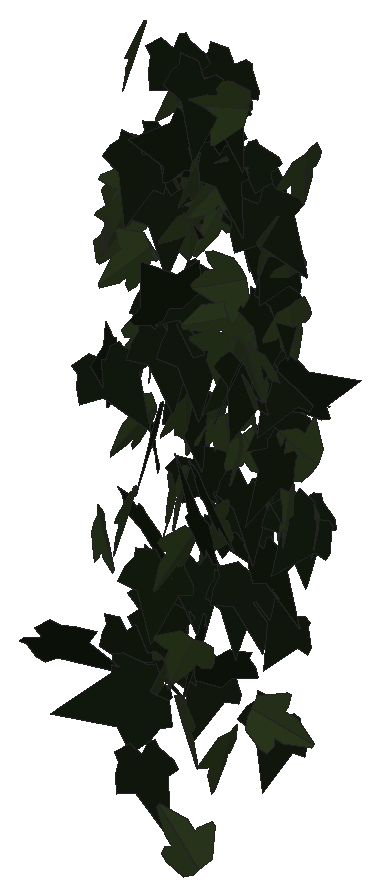
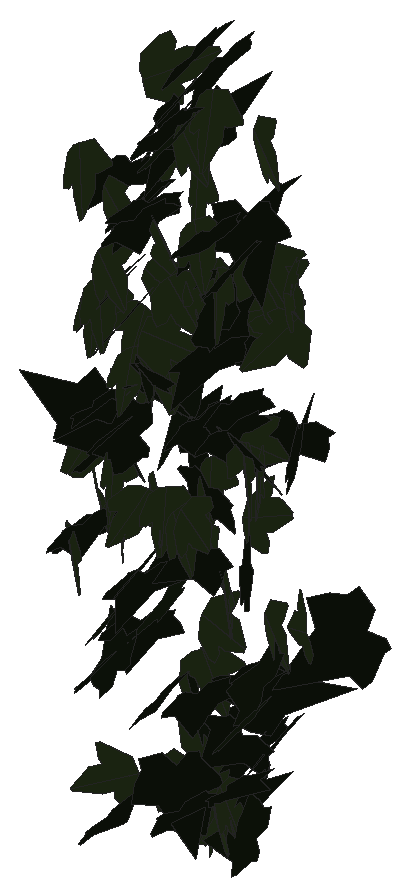
# SketchUp Ruby script. Lengths in inches.
U = 1.inch
M = Sketchup.active_model
def pt(a) = Geom::Point3d.new(a.map { |v| v * U })
def face(e, loops, mat)
  f = e.add_face(loops[0].map { |a| pt(a) })
  loops[1..].each { |l| e.add_face(l.map { |a| pt(a) }).erase! }
  f.material = f.back_material = mat if mat
  f
end
# faces: each face lists its corners as indices into pts; further lists are holes
def faces(e, pts, list, mat = nil) = list.each { |f| face(e, (f[0].is_a?(Array) ? f : [f]).map { |l| l.map { |i| pts[i] } }, mat) }
# xy, xz, yz: faces in a plane at the given z, y or x. An outline is a flat list of corners, or four numbers for a rectangle; further outlines are holes
def ring(l) = l.size == 4 ? [[l[0], l[1]], [l[2], l[1]], [l[2], l[3]], [l[0], l[3]]] : l.each_slice(2).to_a
def flat(e, list, mat, &to3) = list.each { |f| face(e, (f[0].is_a?(Array) ? f : [f]).map { |l| ring(l).map { |u, v| to3.(u, v) } }, mat) }
def xy(e, z, list, mat = nil) = flat(e, list, mat) { |x, y| [x, y, z] }
def xz(e, y, list, mat = nil) = flat(e, list, mat) { |x, z| [x, y, z] }
def yz(e, x, list, mat = nil) = flat(e, list, mat) { |y, z| [x, y, z] }
def lines(e, pts, list) = list.each { |a, b| e.add_line(pt(pts[a]), pt(pts[b])) }
# prism: a flat outline (further loops are holes) pulled along v
def prism(e, loops, v, mat = nil)
  f = face(e, loops, mat); d = Geom::Vector3d.new(v.map { |x| x * U })
  f.pushpull(f.normal.samedirection?(d) ? d.length : -d.length)
end
def box(e, o, s, mat = nil) = prism(e, [[o, [o[0] + s[0], o[1], o[2]], [o[0] + s[0], o[1] + s[1], o[2]], [o[0], o[1] + s[1], o[2]]]], [0, 0, s[2]], mat)
def at(x, y, z, deg = 0) = Geom::Transformation.translation(pt([x, y, z])) * Geom::Transformation.rotation(ORIGIN, Z_AXIS, deg.degrees)
def axes(o, x, y, z) = Geom::Transformation.new([*x, 0, *y, 0, *z, 0, *pt(o).to_a, 1])
def part(name) = M.definitions.add(name)
# library, detail: a bought-in or finely detailed component or shape, given as its bounding box
def library(name, o, s) = part(name).tap { |d| box(d.entities, o, s) }
def detail(e, o, s) = box(e.add_group.entities, o, s)
def put(e, d, t, mat = nil) = e.add_instance(d, t).tap { |i| i.material = mat if mat }
def group(e, t, mat = nil) = e.add_group.tap { |g| g.transformation = t; g.material = mat if mat }.entities
root = M.entities
M.materials.add("efeu1").color = [18, 25, 13]
M.materials.add("efeu2").color = [43, 57, 29]
c1 = part("ivyleaf_10")
p = [[0,0.5,-0.03],[-0.0625,2.02,-0.43],[-0.19,2.01,-0.46],[-0.54,1.05,-0.29],[-0.52,0.625,-0.18],[-0.83,0.76,-0.28],
  [-1.16,0.64,-0.33],[-1.15,0.33,-0.24],[-0.77,-0.39,0.02],[-0.3,-0.51,0.16],[0.04,-0.48,0.23],[-0.02,2.01,-0.4375],
  [-0.06,2.01,-0.43],[0.04,-0.49,0.23],[0.67,-0.49,0.14],[1.38,0.36,-0.2],[1.375,0.51,-0.24],[0.81,0.65,-0.19],
  [0.62,0.59,-0.15],[0.6,1.09,-0.28],[0.5,1.23,-0.31]]
faces(c1.entities,p,[[0,1,2,3,4,5,6,7,8,9,10],[11,12,0,13,14,15,16,17,18,19,20]],"efeu2")
c2 = part("ivyleaf_9")
p = [[1.54,2.16,1.25],[1.36,2.04,1.19],[-0.21,0.99,0.68],[-0.71,1.11,0.82],[-0.85,0.86,0.67],[-0.8,0.17,0.21],
  [-0.9,-0.01,0.1],[-0.67,-0.16,-0.02],[-0.08,-0.08,-0.05],[-0.03,-0.6,-0.4],[0.65,-0.88,-0.66],[0.83,-0.6,-0.49],
  [1.29,-0.42,-0.43],[1.8125,-0.07,-0.26],[1.21,0.44,0.15]]
faces(c2.entities,p,[[0,1,2,3,4,5,6,7,8,9,10,11,12,13,14]],"efeu1")
put(root,c1,axes([556.3125,126.64,275.13],[0.56401,-0.9853,0.35993],[0.15903,-0.32362,-1.13511],[1.03686,0.5856,-0.02169]))
put(root,c2,axes([555.64,127.46,252],[0.64718,-0.92448,0.49192],[0.30397,-0.38755,-1.12823],[1.00212,0.71459,0.02453]))
put(root,c2,axes([556.3,124.88,260.05],[-0.03943,-0.04675,1.18196],[-0.13609,-1.17459,-0.05099],[1.17503,-0.13761,0.03375]))
put(root,c2,axes([556.6,128.28,247.51],[-0.50318,-0.81706,0.39442],[-0.06975,-0.41484,-0.94836],[0.90459,-0.48648,0.14626]))
put(root,c1,axes([556.28,125.15,266.33],[-0.59657,-0.49919,-0.8205],[0.62688,0.52937,-0.77787],[0.72761,-0.86537,-0.00254]))
put(root,c1,axes([556.13,125.17,267.91],[0.21056,-0.52441,1.07679],[0.75537,-0.7903,-0.53259],[0.92946,0.76107,0.1889]))
put(root,c1,axes([556.57,125.68,253.55],[0.52615,-0.98515,0.36041],[0.17062,-0.31747,-1.11685],[1.03504,0.55312,0.0009]))
put(root,c1,axes([556.99,125.87,260.45],[0.40424,-0.52426,-0.91045],[-0.30448,0.8752,-0.63915],[1.00552,0.47579,0.17248]))
put(root,c1,axes([556.09,124.25,252.81],[0.35761,-0.2319,1.0365],[0.97534,-0.36128,-0.41734],[0.42049,1.03522,0.08653]))
put(root,c2,axes([556.02,127.48,245.26],[0.7752,-0.5989,0.50781],[0.39859,-0.31467,-0.97959],[0.67652,0.87165,-0.00473]))
put(root,c1,axes([556.99,124.93,267.99],[-0.02031,-0.99944,0.55469],[0.00222,-0.55481,-0.99957],[1.14305,-0.01668,0.01179]))
put(root,c2,axes([557.23,127.23,262.06],[-1.05217,0.06643,-0.22014],[0.21492,-0.08246,-1.05212],[-0.08175,-1.07179,0.06731]))
put(root,c1,axes([557.22,125.64,269.07],[-0.63028,-0.84539,0.58403],[-0.11789,-0.62113,-1.02631],[1.02072,-0.59375,0.2421]))
put(root,c1,axes([557.16,126.46,261.02],[0.64091,-0.76042,-0.6346],[-0.23557,0.61715,-0.97742],[0.96201,0.65773,0.18344]))
put(root,c2,axes([556.81,127.05,255.54],[-0.4046,0.41446,0.94509],[0.05844,-1.00431,0.46544],[1.03032,0.21972,0.34474]))
put(root,c1,axes([557.2,126.33,261.59],[0.37304,0.66662,-0.89608],[-0.40166,-0.80146,-0.76343],[-1.04212,0.54753,-0.02651]))
put(root,c2,axes([556.9375,127.43,249.51],[-0.09955,-0.87645,0.59303],[0.15035,-0.60132,-0.86346],[1.0475,0.00302,0.18029]))
put(root,c2,axes([556.86,127.77,269.95],[0.2655,-1.08538,0.06413],[0.01067,-0.06341,-1.11737],[1.08722,0.26567,-0.00469]))
put(root,c2,axes([557.11,127.61,262.68],[-0.11286,-1.0882,-0.13553],[0.02533,0.13362,-1.09398],[1.09631,-0.11511,0.01133]))
put(root,c1,axes([557.44,127.375,246.45],[0.16474,-0.9735,0.30647],[0.09722,-0.29406,-0.98633],[1.01596,0.18599,0.04469]))
put(root,c1,axes([557.375,125.68,257.94],[0.09628,-0.37219,1.11823],[0.27094,-1.08492,-0.38443],[1.14698,0.28752,-0.00306]))
put(root,c2,axes([557.87,125.52,270.79],[0.60279,0.64029,-0.79161],[-0.55902,-0.56074,-0.87923],[-0.85095,0.82193,0.01684]))
put(root,c2,axes([557.02,123.64,261.15],[-0.16084,-0.59584,-0.9611],[0.46324,0.85087,-0.60502],[1.03158,-0.47499,0.12184]))
put(root,c2,axes([557.15,124.82,247.8],[0.24998,-1.07113,0.17564],[0.04005,-0.17101,-1.09991],[1.0847,0.25317,0.00014]))
put(root,c1,axes([557.59,127.51,245.57],[0.59434,-0.90486,0.25286],[0.14863,-0.20489,-1.08253],[0.9277,0.61253,0.01143]))
put(root,c2,axes([557.77,126.07,245.24],[-0.22502,-0.61711,0.98012],[-0.35882,-0.91218,-0.65671],[1.10123,-0.42332,-0.01371]))
put(root,c1,axes([557.92,126.375,245.75],[0.44509,-0.9799,0.09472],[0.03724,-0.08711,-1.07624],[0.98376,0.44664,-0.00211]))
put(root,c1,axes([557.97,124.51,266.23],[-0.21681,-0.17831,1.10809],[0.12288,-1.12556,-0.15708],[1.1156,0.08933,0.23265]))
put(root,c2,axes([557.34,119.23,250.14],[1.22806,0.44859,0.46219],[0.43137,0.16613,-1.3074],[-0.47831,1.30159,0.00758]))
put(root,c1,axes([558.21,126.78,268.36],[0.79931,-0.48239,-0.64322],[-0.20259,0.75689,-0.81939],[0.77806,0.69263,0.44743]))
put(root,c2,axes([558.02,124.67,270.8125],[-0.11677,-1.08771,0.36615],[-0.02693,-0.36534,-1.0939],[1.14737,-0.11928,0.01159]))
put(root,c2,axes([558.15,125.9,250.85],[-0.38996,-1.00944,-0.1488],[0.0464,0.14159,-1.08212],[1.01929,-0.39264,-0.00767]))
put(root,c2,axes([557.87,125.95,248.41],[-0.24815,-0.42512,-1.00772],[0.80186,0.63202,-0.46408],[0.7438,-0.82319,0.16411]))
put(root,c1,axes([558.89,125.57,254.54],[0.40704,-0.65288,-0.73768],[-0.35175,0.64924,-0.76869],[0.92017,0.53699,0.03247]))
put(root,c2,axes([557.92,127.3,266.86],[0.14674,-0.48156,1.01776],[0.61545,-0.82516,-0.47917],[0.94285,0.61358,0.15438]))
put(root,c2,axes([558.28,127.41,270.79],[0.25732,-1.02174,-0.43615],[0.00733,0.44925,-1.0481],[1.11091,0.2337,0.10794]))
put(root,c2,axes([558.52,125.94,268.45],[-0.24771,-1.09137,-0.19604],[0.03207,0.19373,-1.11907],[1.10838,-0.24952,-0.01143]))
put(root,c1,axes([559.11,127.04,270.24],[-0.1522,-1.11281,-0.02709],[0.00219,0.02705,-1.12316],[1.11313,-0.15221,-0.00149]))
put(root,c2,axes([558.76,125.5,262.27],[-0.22177,-1.04022,-0.37124],[0.04911,0.36899,-1.06325],[1.10339,-0.2255,-0.0273]))
put(root,c2,axes([558.81,127.35,250.47],[-0.16845,-1.02661,-0.32116],[0.03345,0.31992,-1.04018],[1.07515,-0.1708,-0.01795]))
put(root,c1,axes([559.05,127.64,258.17],[-0.04841,-0.89408,0.60434],[0.20178,-0.60178,-0.87413],[1.06014,0.07371,0.19397]))
put(root,c2,axes([559.23,127.875,245.49],[-0.38874,-1.06838,0.09552],[-0.0348,-0.08898,-1.13691],[1.07208,-0.39029,-0.00227]))
put(root,c1,axes([559.46,127.74,257.78],[0.11033,-1.05731,0.12968],[0.00012,-0.13036,-1.06297],[1.06523,0.10952,-0.01331]))
put(root,c1,axes([559.5,125.63,259.18],[0.05269,-1.05707,-0.36706],[0.01665,0.36817,-1.05787],[1.11886,0.0443,0.03303]))
put(root,c1,axes([559.53,126.03,267.85],[-0.21648,-1.11946,-0.14462],[0.02582,0.14231,-1.14019],[1.12846,-0.21801,-0.00165]))
put(root,c2,axes([558.95,126.61,259.1],[-0.52797,-0.28013,-0.95176],[0.91114,0.28975,-0.59072],[0.39262,-1.04912,0.09099]))
put(root,c1,axes([559.49,125.63,252.64],[0.09184,-0.82512,0.77525],[0.08397,-0.77069,-0.83021],[1.12906,0.12443,-0.00132]))
put(root,c2,axes([559.47,124.67,264.29],[0.50512,0.44437,1.07602],[-0.78128,-0.74017,0.67244],[0.86306,-0.93011,-0.02104]))
put(root,c1,axes([559.86,127.48,267.76],[-0.57232,-0.80064,0.53157],[-0.1343,-0.54599,-0.96695],[0.9516,-0.55858,0.18323]))
put(root,c2,axes([559.14,126.02,264.75],[0.20337,-0.97242,-0.72905],[-0.00249,0.73885,-0.98619],[1.21536,0.16424,0.11997]))
put(root,c1,axes([559.28,125.79,244.57],[-0.71558,0.75391,-0.60071],[0.4061,-0.44273,-1.0394],[-0.87424,-0.82274,0.00887]))
put(root,c2,axes([560.06,127.09,246.68],[0.38264,0.88653,-0.68701],[-0.32498,-0.60711,-0.96444],[-1.07346,0.49981,0.04708]))
put(root,c2,axes([559.375,126.54,261.89],[-0.00036,-1.18226,-0.1288],[-0.01845,0.12879,-1.18212],[1.18911,0.00165,-0.01838]))
put(root,c1,axes([559.68,125.36,255.77],[0.66935,-0.79193,0.26859],[0.20283,-0.18001,-1.03623],[0.81127,0.6984,0.03747]))
put(root,c2,axes([560.41,122.02,247.41],[-0.10183,-0.7318,-1.20891],[-0.18243,-1.19509,0.73881],[-1.40133,0.20876,-0.00833]))
put(root,c1,axes([559.97,125.04,274.68],[-0.12336,-1.1411,-0.43764],[0.10773,0.428,-1.14633],[1.21739,-0.15351,0.0571]))
put(root,c1,axes([560.1,126.46,273.97],[0.17153,-1.09042,0.35447],[0.02946,-0.3541,-1.10356],[1.14621,0.17229,-0.02468]))
put(root,c2,axes([560,123.33,259.74],[-0.60976,0.22528,-0.94837],[0.8475,-0.43012,-0.64708],[-0.48156,-1.04221,0.06205]))
put(root,c2,axes([559.55,126.36,256.15],[-0.11195,-0.22365,-1.09413],[0.69957,0.84308,-0.24391],[0.87048,-0.7063,0.05531]))
put(root,c2,axes([559.91,124.53,276.53],[0.41084,-1.14036,-0.40828],[-0.11352,0.39297,-1.21185],[1.20591,0.4255,0.02502]))
put(root,c2,axes([560.0625,127.9375,274.06],[-0.02921,-0.96271,0.57528],[0.18384,-0.5718,-0.94756],[1.10633,0.0696,0.17264]))
put(root,c1,axes([560.73,124.9,271.09],[0.21692,-0.99031,-0.56397],[-0.06023,0.56333,-1.01236],[1.13805,0.21857,0.05392]))
put(root,c1,axes([560.65,127.02,258.11],[-0.36681,-1.00026,-0.15339],[0.16122,0.10331,-1.05922],[0.99903,-0.38394,0.11461]))
put(root,c2,axes([560.41,127.73,274.6],[-0.16549,-1.1053,0.19456],[-0.0353,-0.19144,-1.1176],[1.12173,-0.16909,-0.00647]))
put(root,c2,axes([560.7,125.32,248.85],[-0.68503,0.32815,-0.78247],[0.72694,-0.29168,-0.75874],[-0.4376,-0.99822,-0.03552]))
put(root,c2,axes([561.02,123.86,272.74],[-0.09089,-0.11257,1.15808],[-0.72882,-0.89998,-0.14468],[0.907,-0.73447,-0.00021]))
put(root,c2,axes([560.56,127.73,249.77],[0.09415,-1.01917,0.23102],[0.0438,-0.22791,-1.02327],[1.0441,0.10146,0.02209]))
put(root,c1,axes([561.48,123.59,249.29],[-0.82836,-0.49623,0.46274],[-0.38542,-0.25688,-0.96541],[0.55841,-0.91341,0.02011]))
put(root,c1,axes([560.43,127.26,269],[0.62028,-0.5236,-0.82353],[0.65692,-0.49759,0.81115],[-0.72169,-0.90297,0.03054]))
put(root,c2,axes([560.72,126.24,253.85],[0.82275,-0.5227,-0.42626],[-0.2102,0.44016,-0.94546],[0.64088,0.8154,0.23712]))
put(root,c1,axes([562.04,125.89,264.21],[-0.30228,-0.1415,1.10941],[-0.84916,-0.71885,-0.32306],[0.72783,-0.89745,0.08385]))
put(root,c2,axes([560.98,121.09,244.91],[0.30715,-1.0927,-0.39439],[-0.06478,0.3912,-1.1343],[1.15989,0.31121,0.04109]))
put(root,c1,axes([561.88,126.24,257.78],[0.37759,-0.60551,-0.88548],[-0.45434,0.7601,-0.71352],[0.97175,0.59067,0.01046]))
put(root,c2,axes([561.84,124.8,273.4],[-0.00972,-0.02449,-1.21503],[-0.82648,0.89096,-0.01135],[0.89098,0.82619,-0.02378]))
put(root,c2,axes([561.4,127.35,254.74],[0.08085,-1.00803,-0.59661],[-0.01357,0.59719,-1.01084],[1.17128,0.07651,0.02947]))
put(root,c1,axes([562.51,125.125,266.35],[0.58599,-0.20604,-1.04989],[-1.00759,0.29634,-0.62054],[0.35985,1.16527,-0.02783]))
put(root,c2,axes([561.55,127.74,270.34],[-0.16033,-1.12703,-0.08932],[0.00069,0.09012,-1.13832],[1.13057,-0.15988,-0.01198]))
put(root,c2,axes([561.34,125.91,274.49],[0.41081,-1.08714,-0.00895],[-0.00125,0.00909,-1.16217],[1.08717,0.41081,0.00204]))
put(root,c2,axes([561.41,127.17,270.83],[0.1075,-0.93748,-0.60834],[0.09572,0.61663,-0.93334],[1.11346,0.0375,0.13897]))
put(root,c1,axes([562.3,125.07,263.22],[-1.07584,-0.43705,0.30582],[-0.2832,-0.11542,-1.16123],[0.45203,-1.11249,0.00034]))
put(root,c2,axes([561.53,127.3,255.2],[0.22439,-1.14973,0.31375],[0.07099,-0.3058,-1.17138],[1.18966,0.2351,0.01072]))
put(root,c2,axes([561.7,124.18,275.89],[0.00162,-1.22118,0.35141],[-0.02208,-0.35139,-1.22099],[1.27055,-0.00454,-0.02166]))
put(root,c1,axes([561.93,126.99,257.65],[-0.5849,-0.70495,-0.56787],[0.54498,0.26561,-0.89106],[0.72279,-0.77073,0.21233]))
put(root,c1,axes([562.45,124.67,244.59],[0.17195,-1.20083,0.0992],[0.02691,-0.09636,-1.21301],[1.20462,0.17356,0.01293]))
put(root,c1,axes([563,124.58,274.91],[-0.19972,-0.14993,-1.19861],[-0.89619,-0.79619,0.24892],[-0.80994,0.91795,0.02013]))
put(root,c1,axes([562.57,123.79,255.25],[0.02085,-0.79247,-0.83201],[0.03532,0.83219,-0.79176],[1.14848,-0.0112,0.03945]))
put(root,c1,axes([562.7,124.32,271.58],[0.11534,0.48889,-1.11409],[-0.35596,-1.05655,-0.5005],[-1.1634,0.37174,0.04269]))
put(root,c2,axes([563.15,125.9375,262.32],[-1.05837,-0.24788,0.07643],[-0.07196,-0.0279,-1.08696],[0.24922,-1.06076,0.01073]))
put(root,c2,axes([562.53,126.22,251.84],[-0.25916,-0.93451,-0.53693],[0.11869,0.52413,-0.96952],[1.07122,-0.28416,-0.02248]))
put(root,c2,axes([562.55,128.19,244.19],[-0.16887,-1.1325,0.35966],[0.0162,-0.36543,-1.14308],[1.18813,-0.15598,0.0667]))
put(root,c1,axes([562.81,126.43,263.18],[-0.20127,-1.05471,-0.20418],[0.30869,0.1422,-1.0388],[1.02899,-0.24896,0.27169]))
put(root,c1,axes([563.01,127.18,259.03],[0.11774,-1.03486,-0.41635],[0.03767,0.42211,-1.03853],[1.11484,0.09503,0.07906]))
put(root,c2,axes([563.12,125.09,262.94],[-0.69701,0.55547,-0.75282],[0.59621,-0.45973,-0.89123],[-0.72099,-0.91717,-0.00921]))
put(root,c2,axes([562.36,127.9,250.66],[0.8301,-0.32,-0.56805],[0.53606,-0.18847,0.88952],[-0.3711,-0.98804,0.0143]))
put(root,c1,axes([562.9375,125.31,261.55],[-0.82438,0.68978,-0.18309],[0.11647,-0.14595,-1.07427],[-0.7041,-0.83176,0.03666]))
put(root,c2,axes([562.25,126.9,260.39],[0.84894,-0.0895,0.67242],[0.67822,0.13362,-0.83847],[-0.01363,1.07471,0.16025]))
put(root,c1,axes([563.19,127.54,267.82],[0.14265,-1.05802,0.31881],[0.01376,-0.31973,-1.06723],[1.10493,0.14057,-0.02787]))
put(root,c1,axes([563.6,125.9375,255.9],[0.06043,0.10332,-1.13934],[-0.49798,1.02955,0.06695],[1.02995,0.49172,0.09922]))
put(root,c2,axes([562.81,126.1875,269.97],[-0.02378,-1.11262,0.11863],[0.00391,-0.11873,-1.11286],[1.11892,-0.02323,0.00641]))
put(root,c2,axes([562.64,124.16,272.61],[0.45489,-1.07791,-0.02188],[-0.00804,0.02035,-1.16996],[1.0781,0.45496,0.0005]))
put(root,c2,axes([563.03,125.54,261.875],[-0.04106,-1.05748,0.55553],[-0.0482,-0.55394,-1.05802],[1.19355,-0.05875,-0.02361]))
put(root,c2,axes([562.9375,125.84,269.42],[0.14319,-1.07328,0.22477],[0.07944,-0.21593,-1.08168],[1.09369,0.1562,0.04914]))
put(root,c2,axes([563.09,127.62,266.65],[-0.20535,-0.8747,0.65751],[0.08237,-0.67944,-0.87816],[1.09116,-0.11332,0.19002]))
put(root,c2,axes([562.92,126.78,252.85],[0.62789,-0.97333,-0.18569],[-0.06447,0.17924,-1.1575],[0.98878,0.62977,0.04244]))
put(root,c1,axes([563.65,127.29,266.24],[-0.12954,-1.12733,-0.11178],[0.02264,0.10991,-1.1347],[1.13263,-0.13113,0.0099]))
put(root,c2,axes([563.7,127.7,259.41],[-0.42087,-0.71799,0.81878],[-0.21202,-0.80699,-0.81662],[1.06816,-0.44307,0.16052]))
put(root,c1,axes([562.98,126.5625,245.17],[0.34313,0.26632,1.05489],[0.86475,0.60449,-0.43389],[-0.66026,0.93012,-0.02006]))
put(root,c2,axes([563.81,127.43,261.3],[-0.43846,-0.9341,0.34741],[-0.09963,-0.33655,-1.03067],[0.99162,-0.44684,0.05005]))
put(root,c2,axes([563.46,126.43,264.47],[0.04376,-1.03229,0.49712],[0.08178,-0.4934,-1.03176],[1.14283,0.07484,0.0548]))
put(root,c2,axes([563.74,127.46,249.79],[-0.26582,-0.89868,0.57094],[-0.01343,-0.58559,-0.92799],[1.06462,-0.23178,0.13085]))
put(root,c2,axes([564.39,120.86,256.39],[0.44101,-0.68015,1.07494],[-0.44856,0.98148,0.80504],[-1.19034,-0.62184,0.09489]))
put(root,c1,axes([564.14,124.33,263.66],[-1.06895,0.26006,-0.05666],[0.05443,-0.01599,-1.10013],[-0.26053,-1.07033,0.00267]))
put(root,c1,axes([564.75,119.6,242.25],[0.85623,0.21164,0.86664],[-0.84988,-0.1717,0.8816],[0.27123,-1.20612,0.02657]))
put(root,c2,axes([563.8125,126.83,265.66],[0.17873,-1.05558,0.29703],[0.08796,-0.28618,-1.06995],[1.09305,0.19563,0.03753]))
put(root,c1,axes([564.59,127.23,271.76],[-0.03361,-1.14125,-0.19402],[0.04718,0.19259,-1.14101],[1.15666,-0.04101,0.04091]))
put(root,c1,axes([564.51,125.46,269.36],[0.37245,-0.95639,0.50622],[0.17301,-0.47585,-1.0263],[1.06818,0.41055,-0.01028]))
put(root,c2,axes([564.47,120.47,259.34],[1.05146,-0.34811,-0.7649],[-0.73068,0.22656,-1.10752],[0.41518,1.28035,-0.01199]))
put(root,c2,axes([564.2,124.83,270.56],[0.1624,-0.87289,-0.80503],[0.21355,0.82075,-0.84685],[1.16808,-0.02869,0.26674]))
put(root,c1,axes([564.73,126.18,265.02],[-0.13584,-1.08628,-0.14102],[0.22919,0.11077,-1.07403],[1.07115,-0.16146,0.21192]))
put(root,c2,axes([564.04,127.32,260.59],[0.16551,-0.06758,1.13669],[1.08701,-0.33275,-0.17806],[0.33916,1.09942,0.01598]))
put(root,c2,axes([565.2,125.02,259.02],[-1.06015,0.03656,-0.45138],[0.44929,-0.05907,-1.06003],[-0.05674,-1.15073,0.04007]))
put(root,c2,axes([564.69,126.95,255.64],[-0.07048,-1.17215,-0.15641],[0.04376,0.15399,-1.17377],[1.18173,-0.07561,0.03414]))
put(root,c1,axes([564.74,125.875,256.49],[0.87862,-0.57215,0.47806],[0.38877,-0.27889,-1.04831],[0.6362,0.96059,-0.01961]))
put(root,c1,axes([565.17,126.73,258.15],[-0.1056,0.91491,0.6919],[0.08561,-0.6866,0.92097],[1.14387,0.13585,-0.00505]))
put(root,c1,axes([565.26,127.03,254.94],[0.68993,-0.7307,-0.37216],[-0.16421,0.35339,-0.99829],[0.80341,0.69973,0.11555]))
put(root,c2,axes([565.25,126.96,255.12],[-0.45032,-0.87896,0.52011],[-0.14636,-0.50702,-0.98355],[1.01077,-0.46501,0.0893]))
